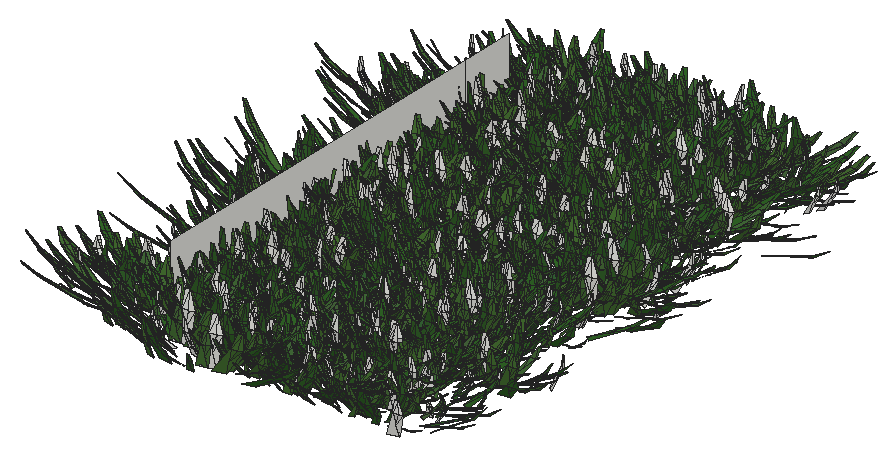
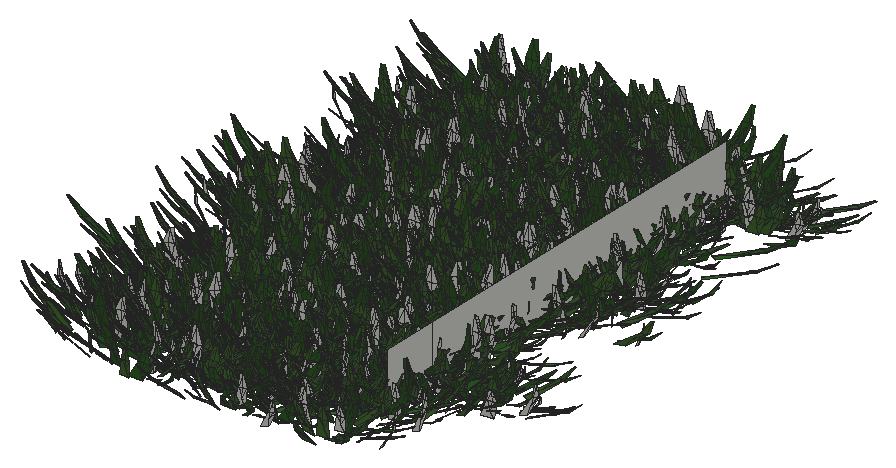
# SketchUp Ruby script. Lengths in inches.
U = 1.inch
M = Sketchup.active_model
def pt(a) = Geom::Point3d.new(a.map { |v| v * U })
def face(e, loops, mat)
  f = e.add_face(loops[0].map { |a| pt(a) })
  loops[1..].each { |l| e.add_face(l.map { |a| pt(a) }).erase! }
  f.material = f.back_material = mat if mat
  f
end
# faces: each face lists its corners as indices into pts; further lists are holes
def faces(e, pts, list, mat = nil) = list.each { |f| face(e, (f[0].is_a?(Array) ? f : [f]).map { |l| l.map { |i| pts[i] } }, mat) }
# xy, xz, yz: faces in a plane at the given z, y or x. An outline is a flat list of corners, or four numbers for a rectangle; further outlines are holes
def ring(l) = l.size == 4 ? [[l[0], l[1]], [l[2], l[1]], [l[2], l[3]], [l[0], l[3]]] : l.each_slice(2).to_a
def flat(e, list, mat, &to3) = list.each { |f| face(e, (f[0].is_a?(Array) ? f : [f]).map { |l| ring(l).map { |u, v| to3.(u, v) } }, mat) }
def xy(e, z, list, mat = nil) = flat(e, list, mat) { |x, y| [x, y, z] }
def xz(e, y, list, mat = nil) = flat(e, list, mat) { |x, z| [x, y, z] }
def yz(e, x, list, mat = nil) = flat(e, list, mat) { |y, z| [x, y, z] }
def lines(e, pts, list) = list.each { |a, b| e.add_line(pt(pts[a]), pt(pts[b])) }
# prism: a flat outline (further loops are holes) pulled along v
def prism(e, loops, v, mat = nil)
  f = face(e, loops, mat); d = Geom::Vector3d.new(v.map { |x| x * U })
  f.pushpull(f.normal.samedirection?(d) ? d.length : -d.length)
end
def box(e, o, s, mat = nil) = prism(e, [[o, [o[0] + s[0], o[1], o[2]], [o[0] + s[0], o[1] + s[1], o[2]], [o[0], o[1] + s[1], o[2]]]], [0, 0, s[2]], mat)
def at(x, y, z, deg = 0) = Geom::Transformation.translation(pt([x, y, z])) * Geom::Transformation.rotation(ORIGIN, Z_AXIS, deg.degrees)
def axes(o, x, y, z) = Geom::Transformation.new([*x, 0, *y, 0, *z, 0, *pt(o).to_a, 1])
def part(name) = M.definitions.add(name)
# library, detail: a bought-in or finely detailed component or shape, given as its bounding box
def library(name, o, s) = part(name).tap { |d| box(d.entities, o, s) }
def detail(e, o, s) = box(e.add_group.entities, o, s)
def put(e, d, t, mat = nil) = e.add_instance(d, t).tap { |i| i.material = mat if mat }
def group(e, t, mat = nil) = e.add_group.tap { |g| g.transformation = t; g.material = mat if mat }.entities
root = M.entities
M.materials.add("Material82").color = [68, 110, 58]
M.materials.add("Material83").color = [48, 90, 38]
M.materials.add("Material84").color = [68, 110, 48]
M.materials.add("Material85").color = [48, 90, 48]
M.materials.add("Material86").color = [58, 110, 58]
M.materials.add("Material87").color = [58, 90, 38]
M.materials.add("Material88").color = [68, 100, 58]
M.materials.add("Material89").color = [48, 100, 38]
c1 = part("grass00")
p = [[-0.6875,0.15,0],[-0.56,0.08,5.52],[-0.04,0.03,2.76],[0.48,-0.02,0],[0.35,-0.02,5.52],[-0.1,-0.14,5.52],
  [-0.12,0.65,8.37],[-0.42,0.65,8.37]]
faces(c1.entities,p,[[0,1,2,3],[3,2,4],[1,5,2],[5,4,2],[1,6,5],[4,5,6],[7,6,1]])
c2 = part("Group16\#1")
put(c2.entities,c1,axes([1.44,-0.61,-0.01],[0.05352,0.12609,0],[-0.10704,0.04543,0.07239],[0.06664,-0.02828,0.11628]),"Material85")
put(c2.entities,c1,axes([0.76,-0.15,-0.01],[0.04676,0.24062,0],[-0.23162,0.04501,0.06642],[0.0652,-0.01267,0.23595]),"Material82")
put(c2.entities,c1,axes([0.79,0.01,-0.01],[-0.00606,0.34651,0],[-0.34381,-0.00602,0.0432],[0.04319,0.00076,0.34386]))
put(c2.entities,c1,axes([1,0.23,-0.01],[-0.07192,0.31144,0],[-0.28722,-0.06632,0.1236],[0.12043,0.02781,0.29478]),"Material84")
put(c2.entities,c1,axes([1.66,0.77,-0.01],[-0.13828,0.29651,0],[-0.21551,-0.1005,0.22471],[0.20365,0.09498,0.23779]),"Material89")
put(c2.entities,c1,axes([0.6875,0.52,-0.01],[-0.18126,0.24051,0],[-0.22746,-0.17142,0.09788],[0.07817,0.05891,0.28481]),"Material84")
put(c2.entities,c1,axes([0.68,0.78,-0.01],[-0.215,0.18688,0],[-0.12385,-0.14248,0.21334],[0.13995,0.16101,0.18878]),"Material82")
put(c2.entities,c1,axes([0.56,1,-0.01],[-0.13756,0.07624,0],[-0.06159,-0.11112,0.0927],[0.04494,0.08108,0.12705]),"Material84")
put(c2.entities,c1,axes([0.2,0.64,-0.01],[-0.23729,0.07254,0],[-0.05711,-0.18681,0.153],[0.04473,0.14632,0.19535]),"Material89")
put(c2.entities,c1,axes([0.0625,0.72,-0.01],[-0.28874,0.02525,0],[-0.02179,-0.24916,0.14647],[0.01276,0.14591,0.25012]),"Material82")
put(c2.entities,c1,axes([-0.08,0.62,-0.01],[-0.34089,-0.04187,0],[0.03255,-0.26504,0.216],[-0.02633,0.21439,0.26703]),"Material89")
put(c2.entities,c1,axes([-0.34,0.98,-0.01],[-0.14314,-0.0493,0],[0.04397,-0.12769,0.06843],[-0.02228,0.0647,0.13505]),"Material89")
put(c2.entities,c1,axes([-0.87,1.45,-0.01],[-0.23488,-0.14114,0],[0.13761,-0.22901,0.06087],[-0.03135,0.05217,0.26717]))
put(c2.entities,c1,axes([-0.72,0.77,-0.01],[-0.14208,-0.13251,0],[0.07209,-0.0773,0.16301],[-0.11118,0.11922,0.1057]),"Material89")
put(c2.entities,c1,axes([-0.62,0.43,-0.01],[-0.14845,-0.21203,0],[0.18654,-0.13061,0.12304],[-0.10079,0.07057,0.22772]),"Material82")
put(c2.entities,c1,axes([-0.68,0.29,-0.01],[-0.13639,-0.32136,0],[0.31723,-0.13464,0.05579],[-0.05136,0.0218,0.34462]),"Material83")
put(c2.entities,c1,axes([-0.64,0.125,-0.01],[-0.0458,-0.23569,0],[0.22124,-0.043,0.08276],[-0.08124,0.01579,0.22538]),"Material86")
put(c2.entities,c1,axes([-1.6,-0.03,-0.01],[0.00576,-0.32897,0],[0.27526,0.00482,0.18018],[-0.18015,-0.00315,0.2753]),"Material84")
put(c2.entities,c1,axes([-1.36,-0.31,-0.01],[0.05718,-0.24765,0],[0.18172,0.04196,0.17267],[-0.16825,-0.03885,0.1865]),"Material89")
put(c2.entities,c1,axes([-1.54,-0.72,-0.01],[0.06537,-0.14017,0],[0.13555,0.06321,0.03939],[-0.0357,-0.01665,0.14956]))
put(c2.entities,c1,axes([-1.19,-0.9,-0.01],[0.09597,-0.12735,0],[0.11214,0.08451,0.07557],[-0.06035,-0.04548,0.14042]),"Material88")
put(c2.entities,c1,axes([-0.47,-0.54,-0.01],[0.11588,-0.10072,0],[0.0618,0.0711,0.12124],[-0.07953,-0.0915,0.0942]))
put(c2.entities,c1,axes([-0.47,-0.84,-0.01],[0.11927,-0.0661,0],[0.06603,0.11913,0.00646],[-0.00313,-0.00565,0.13621]),"Material84")
put(c2.entities,c1,axes([-0.38,-1.24,-0.01],[0.28037,-0.08571,0],[0.0618,0.20215,0.20315],[-0.05939,-0.19428,0.21139]),"Material88")
put(c2.entities,c1,axes([-0.06,-0.66,-0.01],[0.22719,-0.01987,0],[0.01247,0.14255,0.17758],[-0.01547,-0.17691,0.1431]),"Material87")
put(c2.entities,c1,axes([0.11,-0.89,-0.01],[0.14882,0.01828,0],[-0.01058,0.08611,0.12229],[0.01491,-0.12138,0.08676]),"Material85")
put(c2.entities,c1,axes([0.25,-0.72,-0.01],[0.20481,0.07053,0],[-0.06206,0.18022,0.10291],[0.03351,-0.0973,0.1906]),"Material85")
put(c2.entities,c1,axes([0.85,-1.42,-0.01],[0.16481,0.09904,0],[-0.09472,0.15762,0.05616],[0.02893,-0.04814,0.18389]),"Material84")
put(c2.entities,c1,axes([1.01,-1.09,-0.01],[0.21858,0.20385,0],[-0.17495,0.1876,0.15339],[0.10462,-0.11218,0.25652]),"Material89")
put(c2.entities,c1,axes([1.01,-0.71,-0.01],[0.08733,0.12473,0],[-0.06445,0.04512,0.13037],[0.1068,-0.07477,0.07867]),"Material85")
c3 = part("Group15\#1")
put(c3.entities,c2,at(0,0,0))
c4 = part("3darcstudiotree_grass00\#1")
put(c4.entities,c3,at(0,0,0))
yz(root,626.34,[[1000.12,-29.74,1040.81,-23.22],[1040.81,-29.74,1046.93,-23.22]])
put(root,c4,axes([634.17,994.64,-29.74],[1.98347,-1.087,0],[3.74124,1.06175,-0.05142],[0.23843,0.06767,1.97373]))
put(root,c4,axes([640.47,996.4,-29.74],[3.93037,0.00712,0],[-0.01552,1.3324,-0.03904],[-0.00131,0.11261,1.85207]))
put(root,c4,axes([629.9,996.72,-29.74],[1.61856,-1.20753,0],[3.98562,0.83088,-0.05061],[0.25894,0.05398,1.95538]))
put(root,c4,axes([645.26,996.73,-29.74],[3.29344,0.56908,0],[-1.86687,1.68036,-0.0492],[-0.08744,0.0787,1.54416]))
put(root,c4,axes([624.54,997.4,-29.74],[3.81318,-1.10593,0],[2.582,1.38461,-0.02397],[0.05758,0.03088,1.32443]))
put(root,c4,axes([651,996.68,-29.74],[-4.26775,-0.24104,0],[0.59342,-1.63411,-0.00988],[0.00789,-0.02172,1.76639]))
put(root,c4,axes([636.05,997.08,-29.74],[-2.26608,1.33318,0],[-3.11704,-0.82402,-0.02214],[-0.10686,-0.02825,1.63462]))
put(root,c4,axes([645.03,998.28,-29.74],[-0.80049,-1.46058,0],[4.26303,-0.36338,-0.06129],[0.24511,-0.02089,1.3376]))
put(root,c4,axes([650.28,998.75,-29.74],[2.46062,-1.19689,0],[3.08233,0.98555,-0.02965],[0.1062,0.03396,1.3715]))
put(root,c4,axes([641.58,998.23,-29.74],[0.74688,1.42324,0],[-4.33801,0.35406,-0.00233],[-0.01216,0.00099,1.77271]))
put(root,c4,axes([636.44,998.98,-29.74],[0.44293,-1.56057,0],[3.90028,0.17217,-0.04376],[0.2246,0.00991,1.51939]))
put(root,c4,axes([631.02,999.11,-29.74],[-2.26232,-1.46372,0],[3.35674,-0.80691,-0.05337],[0.23381,-0.0562,1.5119]))
put(root,c4,axes([623.73,999.74,-29.74],[3.91343,0.66663,0],[-1.38696,1.26634,-0.02193],[-0.04877,0.04453,1.47013]))
put(root,c4,axes([630.47,1000.89,-29.74],[2.08347,-1.59715,0],[3.15506,0.64012,-0.03693],[0.21917,0.04447,1.77491]))
put(root,c4,axes([623.52,1000.72,-29.74],[-0.96185,1.4826,0],[-3.70839,-0.37418,-0.04208],[-0.21883,-0.02208,1.54007]))
put(root,c4,axes([653.28,1000.91,-29.74],[-0.04598,1.31401,0],[-3.68449,-0.02005,-0.02407],[-0.13013,-0.00071,1.49365]))
put(root,c4,axes([634.63,1000.99,-29.74],[-4.22007,0.35003,0],[-0.86715,-1.62599,-0.01674],[-0.0198,-0.03713,1.81501]))
put(root,c4,axes([641.79,1001.33,-29.74],[-4.17152,-0.5223,0],[1.23744,-1.53711,-0.0262],[0.03523,-0.04376,1.36239]))
put(root,c4,axes([644.3,1001.72,-29.74],[-4.50934,-0.15911,0],[0.38591,-1.70103,-0.03473],[0.01636,-0.07211,1.7157]))
put(root,c4,axes([630.1,1002.77,-29.74],[3.33408,0.32893,0],[-1.10916,1.74856,-0.00744],[-0.00738,0.01164,1.4009]))
put(root,c4,axes([636.5,1003.25,-29.74],[3.70469,-0.86578,0],[1.68851,1.12372,-0.02001],[0.07058,0.04697,1.71774]))
put(root,c4,axes([645.57,1003.15,-29.74],[-2.35898,-1.49879,0],[3.37563,-0.82632,-0.02087],[0.09435,-0.0231,1.58468]))
put(root,c4,axes([642.04,1004.02,-29.74],[3.46997,0.08994,0],[-0.27266,1.63611,-0.01423],[-0.00549,0.03292,1.83161]))
put(root,c4,axes([649.93,1003.53,-29.74],[-3.51315,0.12017,0],[-0.35069,-1.59447,-0.04163],[-0.0224,-0.10183,1.89396]))
put(root,c4,axes([650.12,1004.86,-29.74],[-1.97176,-1.44506,0],[3.679,-0.78074,-0.04084],[0.18174,-0.03857,1.58232]))
put(root,c4,axes([633.3,1005.79,-29.74],[3.27704,0.72692,0],[-1.98468,1.39155,-0.00275],[-0.00611,0.00428,1.37565]))
put(root,c4,axes([639.71,1005.77,-29.74],[4.00271,0.72936,0],[-1.54017,1.31459,-0.00765],[-0.0159,0.01357,1.36419]))
put(root,c4,axes([647.35,1006.16,-29.74],[0.6786,-1.83556,0],[4.57598,0.26311,-0.00277],[0.01184,0.00068,1.49508]))
put(root,c4,axes([628.78,1006.07,-29.74],[-0.56456,1.41966,0],[-3.50259,-0.21664,-0.01794],[-0.10644,-0.00658,1.59592]))
put(root,c4,axes([650.81,1007.01,-29.74],[-0.79088,1.37944,0],[-4.55872,-0.4065,-0.04071],[-0.16308,-0.01454,1.43871]))
put(root,c4,axes([641.16,1007.97,-29.74],[-2.17228,-1.46024,0],[3.41853,-0.79094,-0.03431],[0.15337,-0.03548,1.53951]))
put(root,c4,axes([655.83,1008.1,-29.74],[0.08239,-1.33128,0],[3.65037,0.03514,-0.00377],[0.02295,0.00022,1.66719]))
put(root,c4,axes([629.52,1007.79,-29.74],[0.79004,1.45858,0],[-4.26548,0.35933,-0.00171],[-0.00893,0.00075,1.74655]))
put(root,c4,axes([633.8,1007.79,-29.74],[-4.09965,-0.15274,0],[0.36855,-1.53851,-0.03137],[0.01329,-0.05547,1.3228]))
put(root,c4,axes([644.69,1008.21,-29.74],[2.33704,1.50763,0],[-2.98263,0.71909,-0.02868],[-0.14145,0.0341,1.51486]))
put(root,c4,axes([635.24,1009.36,-29.74],[-2.87872,-0.88154,0],[2.80816,-1.42624,-0.06125],[0.14894,-0.07565,1.36064]))
put(root,c4,axes([628.59,1009.375,-29.74],[-4.49567,-0.3985,0],[0.83225,-1.46029,-0.03373],[0.03467,-0.06083,1.33323]))
put(root,c4,axes([645.99,1009.95,-29.74],[2.20491,1.1875,0],[-2.92266,0.84401,-0.01948],[-0.09978,0.02881,1.72408]))
put(root,c4,axes([640.06,1010.37,-29.74],[2.24844,-1.02464,0],[3.26531,1.11441,-0.03846],[0.14191,0.04843,1.57923]))
put(root,c4,axes([649.77,1010.42,-29.74],[-0.43927,-1.56699,0],[3.3973,-0.14812,-0.00454],[0.02991,-0.0013,1.6986]))
put(root,c4,axes([650.68,1011.78,-29.74],[3.02682,0.57541,0],[-1.48298,1.21327,-0.04063],[-0.10557,0.08637,1.53169]))
put(root,c4,axes([628.51,1011.58,-29.74],[-4.6805,0.28538,0],[-0.54089,-1.37973,-0.03554],[-0.03758,-0.09587,1.83631]))
put(root,c4,axes([636.12,1012.25,-29.74],[-2.16844,-1.41891,0],[2.90956,-0.69156,-0.03107],[0.17396,-0.04135,1.66455]))
put(root,c4,axes([646.55,1012.31,-29.74],[3.34663,1.11106,0],[-2.8307,1.32609,-0.01247],[-0.04541,0.02127,1.86292]))
put(root,c4,axes([640.78,1012.13,-29.74],[0.76665,1.71699,0],[-3.34963,0.23261,-0.02162],[-0.1104,0.00767,1.32159]))
put(root,c4,axes([647.65,1013.62,-29.74],[1.99944,-1.04992,0],[3.08282,0.91308,-0.00267],[0.01382,0.00409,1.87177]))
put(root,c4,axes([650.36,1013.75,-29.74],[3.2382,0.426,0],[-1.27463,1.50694,-0.00681],[-0.01361,0.01609,1.90695]))
put(root,c4,axes([628.09,1013.78,-29.74],[-0.79677,-1.6402,0],[3.36468,-0.25421,-0.01579],[0.08769,-0.00662,1.45182]))
put(root,c4,axes([641.79,1013.5,-29.74],[-3.49855,-0.51529,0],[1.58914,-1.67809,-0.03885],[0.07118,-0.07517,1.78292]))
put(root,c4,axes([634.79,1014.37,-29.74],[0.11814,-1.8536,0],[3.92163,0.03887,-0.05528],[0.30038,0.00298,1.59813]))
put(root,c4,axes([634.25,1015.82,-29.74],[-1.51918,-1.57572,0],[4.39344,-0.65879,-0.02869],[0.10716,-0.01607,1.40786]))
put(root,c4,axes([644.97,1015.89,-29.74],[-1.29023,-1.58759,0],[3.9469,-0.49888,-0.03893],[0.19606,-0.02478,1.64312]))
put(root,c4,axes([642.21,1016.06,-29.74],[-3.86459,-0.0799,0],[0.17825,-1.34085,-0.00586],[0.00206,-0.0155,1.71352]))
put(root,c4,axes([628.06,1015.95,-29.74],[-3.29804,1.27107,0],[-2.52678,-1.01968,-0.01484],[-0.07094,-0.02863,1.85373]))
put(root,c4,axes([624.4,1016.58,-29.74],[3.70183,0.03147,0],[-0.07805,1.42775,-0.0399],[-0.00598,0.10931,1.8861]))
put(root,c4,axes([652.24,1016.74,-29.74],[3.67827,0.2088,0],[-0.57305,1.57009,-0.04848],[-0.0346,0.09479,1.51023]))
put(root,c4,axes([627.24,1018.06,-29.74],[-0.10316,1.55622,0],[-4.09748,-0.04224,-0.03889],[-0.19104,-0.00197,1.50954]))
put(root,c4,axes([624.99,1018.61,-29.74],[-0.3225,-1.34219,0],[4.58247,-0.17125,-0.03587],[0.16603,-0.0062,1.60406]))
put(root,c4,axes([645.23,1018.6,-29.74],[-3.37238,-1.2695,0],[3.05865,-1.2637,-0.04863],[0.19789,-0.08176,1.95701]))
put(root,c4,axes([639.99,1019.23,-29.74],[3.40582,0.10745,0],[-0.34866,1.71886,-0.00093],[-0.00031,0.0015,1.35201]))
put(root,c4,axes([650.6875,1019.08,-29.74],[-1.25158,-1.24653,0],[3.09013,-0.48255,-0.01359],[0.08484,-0.01325,1.67314]))
put(root,c4,axes([633.96,1019.12,-29.74],[-1.65501,1.23077,0],[-2.99443,-0.62625,-0.02105],[-0.13776,-0.02881,1.88169]))
put(root,c4,axes([630.57,1020.41,-29.74],[2.10633,-1.56652,0],[4.07545,0.85227,-0.05067],[0.19625,0.04104,1.51576]))
put(root,c4,axes([649.47,1020.07,-29.74],[-3.55958,-1.14913,0],[2.41323,-1.16263,-0.04086],[0.15936,-0.07677,1.75811]))
put(root,c4,axes([640.49,1020.68,-29.74],[2.63669,-1.45672,0],[3.66232,1.03098,-0.04124],[0.15536,0.04373,1.56101]))
put(root,c4,axes([634,1020.17,-29.74],[-1.69964,1.49974,0],[-3.25198,-0.57319,-0.0353],[-0.21623,-0.03811,1.79152]))
put(root,c4,axes([645.01,1021.25,-29.74],[-3.5162,-0.01544,0],[0.03762,-1.33225,-0.02017],[0.00158,-0.05579,1.77597]))
put(root,c4,axes([628.1875,1022.61,-29.74],[2.48968,-1.1461,0],[2.93182,0.99053,-0.00664],[0.0258,0.00872,1.48048]))
put(root,c4,axes([640.06,1022.29,-29.74],[-0.28743,1.31478,0],[-4.42266,-0.15037,-0.00545],[-0.03167,-0.00108,1.93955]))
put(root,c4,axes([624.54,1022.93,-29.74],[3.82293,-1.07301,0],[2.00012,1.10831,-0.02041],[0.08948,0.04958,1.95445]))
put(root,c4,axes([653.35,1023.46,-29.74],[1.80491,-1.57701,0],[4.14536,0.7379,-0.03311],[0.16907,0.03009,1.9099]))
put(root,c4,axes([636.15,1023.57,-29.74],[-1.1098,-1.31734,0],[3.29231,-0.43138,-0.00285],[0.02011,-0.00264,1.93438]))
put(root,c4,axes([647.56,1023.23,-29.74],[-3.77729,0.83126,0],[-1.83032,-1.29355,-0.03544],[-0.09552,-0.06751,1.55733]))
put(root,c4,axes([641.54,1024.77,-29.74],[0.50947,-1.51274,0],[4.49668,0.23554,-0.03191],[0.15996,0.00838,1.71939]))
put(root,c4,axes([633.26,1025.21,-29.74],[-3.21191,1.28173,0],[-2.59769,-1.01243,-0.03007],[-0.15402,-0.06003,1.97134]))
put(root,c4,axes([650.1,1025.53,-29.74],[-2.97894,1.37787,0],[-2.78264,-0.93567,-0.01811],[-0.06538,-0.02199,1.30017]))
put(root,c4,axes([647.82,1025.7,-29.74],[-3.83744,0.33373,0],[-0.9251,-1.65441,-0.02531],[-0.02998,-0.05361,1.77094]))
put(root,c4,axes([628.76,1026.02,-29.74],[1.96349,1.64722,0],[-3.56633,0.66117,-0.03464],[-0.18907,0.03505,1.78143]))
put(root,c4,axes([653.125,1027.18,-29.74],[1.28722,-1.76401,0],[4.46987,0.50729,-0.04991],[0.26732,0.03034,1.94306]))
put(root,c4,axes([655.39,1026.63,-29.74],[-1.91663,1.65988,0],[-3.0087,-0.54032,-0.04508],[-0.21948,-0.03942,1.32557]))
put(root,c4,axes([629.63,1027.125,-29.74],[-1.20508,-1.27416,0],[3.97727,-0.58504,-0.0406],[0.22085,-0.03249,1.84742]))
put(root,c4,axes([644.97,1027.625,-29.74],[0.71095,-1.43364,0],[4.62721,0.35689,-0.06032],[0.23627,0.01822,1.41053]))
put(root,c4,axes([640.83,1028.21,-29.74],[-4.16983,-0.88311,0],[1.85574,-1.3628,-0.02099],[0.05036,-0.03698,1.49075]))
put(root,c4,axes([636.35,1028.125,-29.74],[-3.85239,-0.20163,0],[0.58764,-1.74619,-0.01228],[0.0079,-0.02349,1.63767]))
put(root,c4,axes([645.87,1028.78,-29.74],[3.70622,-0.07941,0],[0.19617,1.42399,-0.02262],[0.0073,0.05302,1.6131]))
put(root,c4,axes([640.81,1029.1,-29.74],[-1.93961,-1.1589,0],[2.81158,-0.73187,-0.03406],[0.19491,-0.05074,1.73123]))
put(root,c4,axes([652.19,1029.82,-29.74],[0.12202,-1.72029,0],[4.34373,0.04792,-0.00421],[0.02346,0.00026,1.81536]))
put(root,c4,axes([636.4,1029.31,-29.74],[-1.66799,1.12199,0],[-3.57556,-0.82672,-0.01566],[-0.07039,-0.01628,1.61828]))
put(root,c4,axes([631.24,1030.15,-29.74],[1.69514,-1.26112,0],[3.85825,0.80658,-0.01977],[0.09529,0.01992,1.78562]))
put(root,c4,axes([646.51,1031.72,-29.74],[-0.8203,-1.58295,0],[4.36315,-0.35165,-0.03636],[0.17472,-0.01408,1.63697]))
put(root,c4,axes([651.75,1031.5,-29.74],[-4.26886,-0.01451,0],[0.03771,-1.72573,-0.00939],[0.00047,-0.02147,1.9024]))
put(root,c4,axes([640.88,1031.88,-29.74],[3.91894,1.05311,0],[-2.36552,1.3691,-0.06012],[-0.14517,0.08402,1.3502]))
put(root,c4,axes([633.21,1032.22,-29.74],[3.33812,-0.00931,0],[0.03014,1.68097,-0.0442],[0.00131,0.07293,1.33678]))
put(root,c4,axes([631.17,1032.4,-29.74],[-2.43659,-1.39628,0],[3.54139,-0.96116,-0.05298],[0.19991,-0.05426,1.4759]))
put(root,c4,axes([628.39,1033.15,-29.74],[-3.06856,1.30795,0],[-2.89535,-1.05647,-0.0352],[-0.142,-0.05181,1.62511]))
put(root,c4,axes([640.8125,1033.87,-29.74],[0.60137,-1.69863,0],[3.35822,0.18491,-0.0384],[0.22932,0.01263,1.53253]))
put(root,c4,axes([633.41,1033.97,-29.74],[-0.2328,1.40639,0],[-3.78045,-0.09733,-0.01044],[-0.05523,-0.00142,1.50484]))
put(root,c4,axes([649.28,1034.41,-29.74],[-0.96459,1.39728,0],[-4.50708,-0.48391,-0.06593],[-0.29103,-0.03125,1.60187]))
put(root,c4,axes([647.625,1034.51,-29.74],[0.06651,1.49398,0],[-4.62108,0.032,-0.00579],[-0.03066,0.00021,1.83497]))
put(root,c4,axes([644.61,1035.59,-29.74],[3.81628,-0.13918,0],[0.37321,1.59155,-0.00914],[0.00528,0.02252,1.90465]))
put(root,c4,axes([640.98,1035.87,-29.74],[-1.5249,1.25696,0],[-3.62628,-0.68422,-0.02774],[-0.1175,-0.02217,1.41462]))
put(root,c4,axes([633.98,1035.92,-29.74],[-1.7842,1.38137,0],[-4.14651,-0.83297,-0.01882],[-0.07173,-0.01441,1.49212]))
put(root,c4,axes([627.18,1036.78,-29.74],[-1.63198,-1.29559,0],[3.66951,-0.7189,-0.01655],[0.08632,-0.01691,1.78815]))
put(root,c4,axes([651.8,1036.6,-29.74],[-0.60649,1.78928,0],[-3.60415,-0.19,-0.04319],[-0.29403,-0.0155,1.87209]))
put(root,c4,axes([640.23,1037.8125,-29.74],[3.33503,1.17525,0],[-2.6851,1.18507,-0.00121],[-0.00399,0.00176,1.48985]))
put(root,c4,axes([651.26,1038.03,-29.74],[-1.50368,1.17097,0],[-3.52829,-0.70467,-0.03106],[-0.12382,-0.02473,1.32443]))
put(root,c4,axes([644.66,1038.73,-29.74],[0.14571,-1.35454,0],[4.55175,0.07615,-0.04061],[0.20314,0.0034,1.70991]))
put(root,c4,axes([623.48,1038.85,-29.74],[2.90846,1.13793,0],[-2.61613,1.03996,-0.02475],[-0.10205,0.04057,1.62992]))
put(root,c4,axes([627.28,1039,-29.74],[0.65055,1.72425,0],[-3.43127,0.20135,-0.01524],[-0.11013,0.00646,1.90022]))
put(root,c4,axes([635.94,1039,-29.74],[-2.50108,0.95556,0],[-2.98511,-1.21518,-0.02879],[-0.10959,-0.04461,1.7592]))
put(root,c4,axes([623.59,1039.85,-29.74],[4.3644,0.14123,0],[-0.27589,1.32601,-0.01884],[-0.00836,0.04017,1.37151]))
put(root,c4,axes([633.59,1039.84,-29.74],[-0.81871,-1.45227,0],[3.80429,-0.33355,-0.01455],[0.06635,-0.00582,1.36448]))
put(root,c4,axes([653.19,1040.27,-29.74],[3.40778,-1.13854,0],[2.78991,1.29874,-0.02128],[0.06823,0.03176,1.60475]))
put(root,c4,axes([631.21,1040.36,-29.74],[1.18703,1.24458,0],[-3.56072,0.52819,-0.04913],[-0.2933,0.04351,1.81865]))
put(root,c4,axes([638.97,1040.91,-29.74],[4.2261,-0.33522,0],[0.81524,1.59847,-0.02659],[0.0257,0.05039,1.51897]))
put(root,c4,axes([645.72,1041.3125,-29.74],[-4.64372,0.01964,0],[-0.04703,-1.72937,-0.01941],[-0.00122,-0.04491,1.92834]))
put(root,c4,axes([635.77,1042.34,-29.74],[0.27542,-1.59187,0],[4.66457,0.12552,-0.02398],[0.0893,0.0024,1.30813]))
put(root,c4,axes([628.34,1042.02,-29.74],[-3.57616,-1.16474,0],[2.7999,-1.33704,-0.02974],[0.0776,-0.03706,1.35064]))
put(root,c4,axes([645.7,1042.93,-29.74],[4.39151,-0.30239,0],[0.81207,1.8342,-0.04063],[0.02885,0.06516,1.46079]))
put(root,c4,axes([639.65,1042.89,-29.74],[0.23544,-1.60034,0],[3.90526,0.08936,-0.02273],[0.11635,0.00266,1.50351]))
put(root,c4,axes([651.4,1043.24,-29.74],[2.16016,-1.57069,0],[3.42867,0.73339,-0.01711],[0.07383,0.01579,1.43496]))
put(root,c4,axes([628.83,1044.58,-29.74],[3.96997,0.02835,0],[-0.08063,1.7564,-0.04973],[-0.00512,0.11159,1.89995]))
put(root,c4,axes([634.17,1044.57,-29.74],[-3.18032,-1.25414,0],[2.9494,-1.16324,-0.05204],[0.20858,-0.08226,1.77215]))
put(root,c4,axes([639.77,1044.68,-29.74],[3.671,0.98063,0],[-2.61565,1.5229,-0.02464],[-0.07837,0.04563,1.98292]))
put(root,c4,axes([644.28,1045.12,-29.74],[3.22571,-1.00591,0],[2.69072,1.34198,-0.01988],[0.07446,0.03714,1.96304]))
put(root,c4,axes([650.64,1045.67,-29.74],[-1.03876,-1.58927,0],[3.98467,-0.40506,-0.01269],[0.06748,-0.00686,1.69312]))
put(root,c4,axes([627.89,1046.54,-29.74],[2.6716,0.78375,0],[-2.01413,1.06781,-0.0148],[-0.06741,0.03574,1.93047]))
put(root,c4,axes([632.85,1046.79,-29.74],[-4.17606,0.09309,0],[-0.21865,-1.52546,-0.00256],[-0.00085,-0.00591,1.70382]))
put(root,c4,axes([638.3,1047.54,-29.74],[-3.25209,-0.85971,0],[2.35344,-1.3846,-0.05337],[0.14871,-0.08749,1.58535]))
put(root,c4,axes([653,1047.75,-29.74],[-2.22741,-1.08823,0],[2.74712,-0.87452,-0.02577],[0.11865,-0.03777,1.56591]))
put(root,c4,axes([645.32,1047.5,-29.74],[-3.60513,-0.15499,0],[0.46196,-1.67121,-0.01401],[0.00822,-0.02974,1.72979]))
put(root,c4,axes([652.87,1048.46,-29.74],[-2.63384,-1.55649,0],[3.02127,-0.79514,-0.04802],[0.24921,-0.06559,1.69851]))
put(root,c4,axes([634.42,1048.55,-29.74],[-0.69591,-1.28996,0],[3.84518,-0.32263,-0.04713],[0.24772,-0.02078,1.58351]))
put(root,c4,axes([647.75,1048.65,-29.74],[4.30833,-0.24109,0],[0.6166,1.71371,-0.05794],[0.04515,0.12549,1.82474]))
put(root,c4,axes([630.56,1049.1,-29.74],[3.37733,-0.03199,0],[0.10215,1.67739,-0.04057],[0.00409,0.06713,1.33829]))
put(root,c4,axes([639.375,1049.92,-29.74],[-3.50198,-0.71469,0],[1.86103,-1.41828,-0.02021],[0.05866,-0.0447,1.91641]))
put(root,c4,axes([652.53,1050.91,-29.74],[2.75838,0.79761,0],[-2.27657,1.22449,-0.01003],[-0.02813,0.01513,1.36834]))
put(root,c4,axes([645.66,1050.65,-29.74],[-1.99433,1.44629,0],[-3.30766,-0.70937,-0.03157],[-0.17706,-0.03797,1.80167]))
put(root,c4,axes([641.13,1051.35,-29.74],[3.4743,0.19553,0],[-0.61359,1.69568,-0.03434],[-0.02545,0.07034,1.70799]))
put(root,c4,axes([635.35,1050.96,-29.74],[-4.09244,0.60833,0],[-1.31907,-1.38013,-0.00238],[-0.00395,-0.00413,1.31717]))
put(root,c4,axes([629.16,1052.08,-29.74],[1.23256,1.36805,0],[-3.36714,0.47182,-0.0026],[-0.01342,0.00188,1.46428]))
put(root,c4,axes([638.98,1053.15,-29.74],[2.94498,0.60485,0],[-2.04543,1.54892,-0.0178],[-0.03241,0.02454,1.30843]))
put(root,c4,axes([650.41,1053.375,-29.74],[-4.3017,0.59676,0],[-1.104,-1.2377,-0.00518],[-0.01285,-0.0144,1.86492]))
